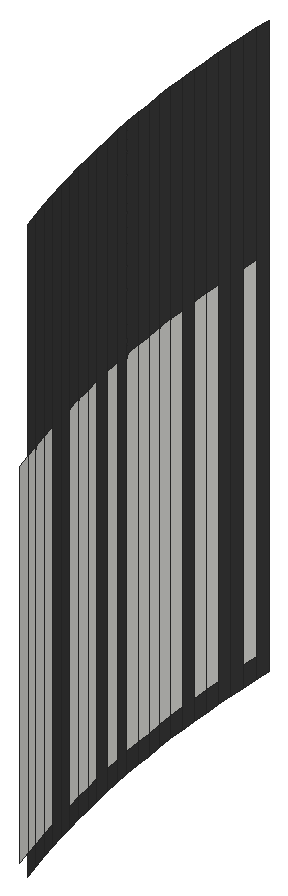
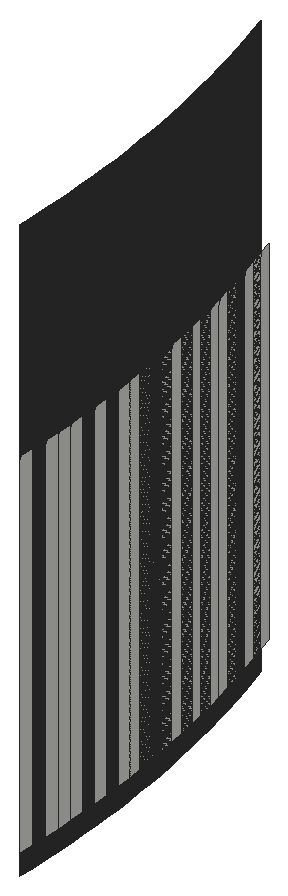
# SketchUp Ruby script. Lengths in inches.
U = 1.inch
M = Sketchup.active_model
def pt(a) = Geom::Point3d.new(a.map { |v| v * U })
def face(e, loops, mat)
  f = e.add_face(loops[0].map { |a| pt(a) })
  loops[1..].each { |l| e.add_face(l.map { |a| pt(a) }).erase! }
  f.material = f.back_material = mat if mat
  f
end
# faces: each face lists its corners as indices into pts; further lists are holes
def faces(e, pts, list, mat = nil) = list.each { |f| face(e, (f[0].is_a?(Array) ? f : [f]).map { |l| l.map { |i| pts[i] } }, mat) }
# xy, xz, yz: faces in a plane at the given z, y or x. An outline is a flat list of corners, or four numbers for a rectangle; further outlines are holes
def ring(l) = l.size == 4 ? [[l[0], l[1]], [l[2], l[1]], [l[2], l[3]], [l[0], l[3]]] : l.each_slice(2).to_a
def flat(e, list, mat, &to3) = list.each { |f| face(e, (f[0].is_a?(Array) ? f : [f]).map { |l| ring(l).map { |u, v| to3.(u, v) } }, mat) }
def xy(e, z, list, mat = nil) = flat(e, list, mat) { |x, y| [x, y, z] }
def xz(e, y, list, mat = nil) = flat(e, list, mat) { |x, z| [x, y, z] }
def yz(e, x, list, mat = nil) = flat(e, list, mat) { |y, z| [x, y, z] }
def lines(e, pts, list) = list.each { |a, b| e.add_line(pt(pts[a]), pt(pts[b])) }
# prism: a flat outline (further loops are holes) pulled along v
def prism(e, loops, v, mat = nil)
  f = face(e, loops, mat); d = Geom::Vector3d.new(v.map { |x| x * U })
  f.pushpull(f.normal.samedirection?(d) ? d.length : -d.length)
end
def box(e, o, s, mat = nil) = prism(e, [[o, [o[0] + s[0], o[1], o[2]], [o[0] + s[0], o[1] + s[1], o[2]], [o[0], o[1] + s[1], o[2]]]], [0, 0, s[2]], mat)
def at(x, y, z, deg = 0) = Geom::Transformation.translation(pt([x, y, z])) * Geom::Transformation.rotation(ORIGIN, Z_AXIS, deg.degrees)
def axes(o, x, y, z) = Geom::Transformation.new([*x, 0, *y, 0, *z, 0, *pt(o).to_a, 1])
def part(name) = M.definitions.add(name)
# library, detail: a bought-in or finely detailed component or shape, given as its bounding box
def library(name, o, s) = part(name).tap { |d| box(d.entities, o, s) }
def detail(e, o, s) = box(e.add_group.entities, o, s)
def put(e, d, t, mat = nil) = e.add_instance(d, t).tap { |i| i.material = mat if mat }
def group(e, t, mat = nil) = e.add_group.tap { |g| g.transformation = t; g.material = mat if mat }.entities
root = M.entities
M.materials.add("1496 AP 8293 CARBON COPY").color = [58, 58, 58]
yz(root,14,[[114.61,129.5,115,138]])
yz(root,14,[[114.61,129,115,143]],"1496 AP 8293 CARBON COPY")
p = [[15.35,106.1,129],[15.24,106.48,129],[15.24,106.48,143],[15.35,106.1,143],[15.125,106.86,129],[15.125,106.86,143],
  [15.02,107.24,129],[15.02,107.24,143],[14.92,107.62,129],[14.92,107.62,143],[14.83,108,129],[14.83,108,143],
  [14.74,108.38,129],[14.74,108.38,143],[14.66,108.76,129],[14.66,108.76,143],[14.58,109.15,129],[14.58,109.15,143],
  [14.5,109.53,129],[14.5,109.53,143],[14.43,109.92,129],[14.43,109.92,143],[14.37,110.31,129],[14.37,110.31,143],
  [14.31,110.7,129],[14.31,110.7,143],[14.26,111.08,129],[14.26,111.08,143],[14.21,111.47,129],[14.21,111.47,143],
  [14.16,111.86,129],[14.16,111.86,143],[14.125,112.25,129],[14.125,112.25,143],[14.09,112.65,129],[14.09,112.65,143],
  [14.0625,113.04,129],[14.0625,113.04,143],[14.04,113.43,129],[14.04,113.43,143],[14.02,113.82,129],[14.02,113.82,143],
  [14.01,114.21,129],[14.01,114.21,143],[14,114.61,129],[14,114.61,143],[15.47,105.73,138],[15.35,106.1,138],
  [15.35,106.1,129.5],[15.47,105.73,129.5],[15.24,106.48,138],[15.24,106.48,129.5],[15.125,106.86,138],[15.125,106.86,129.5],
  [15.02,107.24,138],[15.02,107.24,129.5],[14.92,107.62,138],[14.92,107.62,129.5],[14.83,108,138],[14.83,108,129.5],
  [14.74,108.38,138],[14.74,108.38,129.5],[14.66,108.76,138],[14.66,108.76,129.5],[14.58,109.15,138],[14.58,109.15,129.5],
  [14.5,109.53,138],[14.5,109.53,129.5],[14.43,109.92,138],[14.43,109.92,129.5],[14.37,110.31,138],[14.37,110.31,129.5],
  [14.31,110.7,138],[14.31,110.7,129.5],[14.26,111.08,138],[14.26,111.08,129.5],[14.21,111.47,138],[14.21,111.47,129.5],
  [14.16,111.86,138],[14.16,111.86,129.5],[14.125,112.25,138],[14.125,112.25,129.5],[14.09,112.65,138],[14.09,112.65,129.5],
  [14.0625,113.04,138],[14.0625,113.04,129.5],[14.04,113.43,138],[14.04,113.43,129.5],[14.02,113.82,138],[14.02,113.82,129.5],
  [14.01,114.21,138],[14.01,114.21,129.5],[14,114.61,138],[14,114.61,129.5]]
faces(root,p,[[0,1,2,3],[1,4,5,2],[4,6,7,5],[6,8,9,7],[8,10,11,9],[10,12,13,11],[12,14,15,13],[14,16,17,15],
  [16,18,19,17],[18,20,21,19],[20,22,23,21],[22,24,25,23],[24,26,27,25],[26,28,29,27],[28,30,31,29],[30,32,33,31],
  [32,34,35,33],[34,36,37,35],[36,38,39,37],[38,40,41,39],[40,42,43,41],[42,44,45,43]],"1496 AP 8293 CARBON COPY")
faces(root,p,[[46,47,48,49],[47,50,51,48],[50,52,53,51],[52,54,55,53],[54,56,57,55],[56,58,59,57],[58,60,61,59],[60,62,63,61],
  [62,64,65,63],[64,66,67,65],[66,68,69,67],[68,70,71,69],[70,72,73,71],[72,74,75,73],[74,76,77,75],[76,78,79,77],
  [78,80,81,79],[80,82,83,81],[82,84,85,83],[84,86,87,85],[86,88,89,87],[88,90,91,89],[90,92,93,91]])
